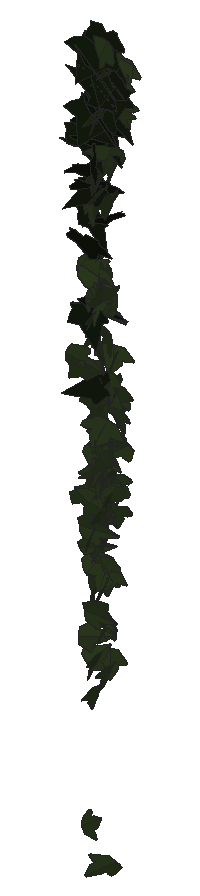
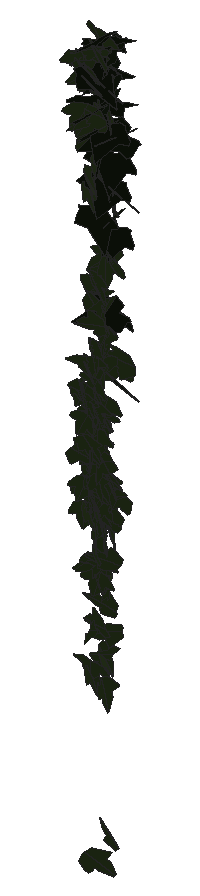
# SketchUp Ruby script. Lengths in inches.
U = 1.inch
M = Sketchup.active_model
def pt(a) = Geom::Point3d.new(a.map { |v| v * U })
def face(e, loops, mat)
  f = e.add_face(loops[0].map { |a| pt(a) })
  loops[1..].each { |l| e.add_face(l.map { |a| pt(a) }).erase! }
  f.material = f.back_material = mat if mat
  f
end
# faces: each face lists its corners as indices into pts; further lists are holes
def faces(e, pts, list, mat = nil) = list.each { |f| face(e, (f[0].is_a?(Array) ? f : [f]).map { |l| l.map { |i| pts[i] } }, mat) }
# xy, xz, yz: faces in a plane at the given z, y or x. An outline is a flat list of corners, or four numbers for a rectangle; further outlines are holes
def ring(l) = l.size == 4 ? [[l[0], l[1]], [l[2], l[1]], [l[2], l[3]], [l[0], l[3]]] : l.each_slice(2).to_a
def flat(e, list, mat, &to3) = list.each { |f| face(e, (f[0].is_a?(Array) ? f : [f]).map { |l| ring(l).map { |u, v| to3.(u, v) } }, mat) }
def xy(e, z, list, mat = nil) = flat(e, list, mat) { |x, y| [x, y, z] }
def xz(e, y, list, mat = nil) = flat(e, list, mat) { |x, z| [x, y, z] }
def yz(e, x, list, mat = nil) = flat(e, list, mat) { |y, z| [x, y, z] }
def lines(e, pts, list) = list.each { |a, b| e.add_line(pt(pts[a]), pt(pts[b])) }
# prism: a flat outline (further loops are holes) pulled along v
def prism(e, loops, v, mat = nil)
  f = face(e, loops, mat); d = Geom::Vector3d.new(v.map { |x| x * U })
  f.pushpull(f.normal.samedirection?(d) ? d.length : -d.length)
end
def box(e, o, s, mat = nil) = prism(e, [[o, [o[0] + s[0], o[1], o[2]], [o[0] + s[0], o[1] + s[1], o[2]], [o[0], o[1] + s[1], o[2]]]], [0, 0, s[2]], mat)
def at(x, y, z, deg = 0) = Geom::Transformation.translation(pt([x, y, z])) * Geom::Transformation.rotation(ORIGIN, Z_AXIS, deg.degrees)
def axes(o, x, y, z) = Geom::Transformation.new([*x, 0, *y, 0, *z, 0, *pt(o).to_a, 1])
def part(name) = M.definitions.add(name)
# library, detail: a bought-in or finely detailed component or shape, given as its bounding box
def library(name, o, s) = part(name).tap { |d| box(d.entities, o, s) }
def detail(e, o, s) = box(e.add_group.entities, o, s)
def put(e, d, t, mat = nil) = e.add_instance(d, t).tap { |i| i.material = mat if mat }
def group(e, t, mat = nil) = e.add_group.tap { |g| g.transformation = t; g.material = mat if mat }.entities
root = M.entities
M.materials.add("1026 AP 7946 SUNNY SIDE UP").color = [254, 231, 186]
M.materials.add("efeu1").color = [18, 25, 13]
M.materials.add("efeu2").color = [43, 57, 29]
c1 = part("ivyleaf_9")
p = [[1.54,2.16,1.25],[1.36,2.04,1.19],[-0.21,0.99,0.68],[-0.71,1.11,0.82],[-0.85,0.86,0.67],[-0.8,0.17,0.21],
  [-0.9,-0.01,0.1],[-0.67,-0.16,-0.02],[-0.08,-0.08,-0.05],[-0.03,-0.6,-0.4],[0.65,-0.88,-0.66],[0.83,-0.6,-0.49],
  [1.29,-0.42,-0.43],[1.8125,-0.07,-0.26],[1.21,0.44,0.15]]
faces(c1.entities,p,[[0,1,2,3,4,5,6,7,8,9,10,11,12,13,14]],"efeu1")
c2 = part("ivyleaf_10")
p = [[0,0.5,-0.03],[-0.0625,2.02,-0.43],[-0.19,2.01,-0.46],[-0.54,1.05,-0.29],[-0.52,0.625,-0.18],[-0.83,0.76,-0.28],
  [-1.16,0.64,-0.33],[-1.15,0.33,-0.24],[-0.77,-0.39,0.02],[-0.3,-0.51,0.16],[0.04,-0.48,0.23],[-0.02,2.01,-0.4375],
  [-0.06,2.01,-0.43],[0.04,-0.49,0.23],[0.67,-0.49,0.14],[1.38,0.36,-0.2],[1.375,0.51,-0.24],[0.81,0.65,-0.19],
  [0.62,0.59,-0.15],[0.6,1.09,-0.28],[0.5,1.23,-0.31]]
faces(c2.entities,p,[[0,1,2,3,4,5,6,7,8,9,10],[11,12,0,13,14,15,16,17,18,19,20]],"efeu2")
put(root,c1,axes([100.36,212.83,266.07],[0.33529,0.09717,-0.0854],[-0.10279,-0.05681,-0.24056],[-0.1732,0.22183,-0.02256]),"1026 AP 7946 SUNNY SIDE UP")
put(root,c2,axes([100.24,212.86,257.25],[-0.07001,-0.03539,0.18134],[0.17886,0.13359,0.05905],[-0.23398,0.1127,-0.00912]),"1026 AP 7946 SUNNY SIDE UP")
put(root,c2,axes([100.12,212.65,261.24],[-0.04534,-0.00324,-0.24949],[0.33942,-0.1109,-0.0256],[-0.17264,-0.21719,0.01519]),"1026 AP 7946 SUNNY SIDE UP")
put(root,c2,axes([100.23,212.86,251.5625],[0.15354,-0.11194,-0.14231],[0.15962,-0.09341,0.15206],[-0.22859,-0.14041,0.01059]),"1026 AP 7946 SUNNY SIDE UP")
put(root,c2,axes([100.43,212.78,258.9375],[0.16208,-0.18655,-0.02128],[-0.02221,0.01458,-0.21941],[0.2941,0.10391,-0.00484]),"1026 AP 7946 SUNNY SIDE UP")
put(root,c1,axes([100.23,212.74,265.85],[0.04431,-0.22984,-0.03374],[0.05092,0.03182,-0.24464],[0.38984,0.02197,0.03579]),"1026 AP 7946 SUNNY SIDE UP")
put(root,c2,axes([100.26,212.65,258.45],[-0.21018,-0.0282,-0.13125],[0.21154,-0.00791,-0.13329],[0.02448,-0.17381,0.02487]),"1026 AP 7946 SUNNY SIDE UP")
put(root,c1,axes([100.51,213.08,267.23],[0.001,0.16822,-0.15884],[0.00207,-0.15056,-0.18219],[-0.38323,-0.00038,-0.0014]),"1026 AP 7946 SUNNY SIDE UP")
put(root,c2,axes([100.24,213.1,262.17],[0.07325,-0.045,0.17694],[0.23261,-0.0942,-0.06684],[0.17607,0.14317,0.01469]),"1026 AP 7946 SUNNY SIDE UP")
put(root,c1,axes([100.45,212.58,265.3125],[0.16525,0.2139,-0.01562],[-0.01271,-0.01569,-0.25181],[-0.36408,0.09763,0.0017]),"1026 AP 7946 SUNNY SIDE UP")
put(root,c2,axes([100.375,212.94,260.22],[0.19343,-0.13157,0.05993],[0.05347,-0.04896,-0.18684],[0.23795,0.11796,-0.00673]),"1026 AP 7946 SUNNY SIDE UP")
put(root,c2,axes([100.375,212.87,262.48],[0.04091,0.22554,0.05224],[-0.00783,0.05028,-0.23335],[-0.36297,0.02433,0.01092]),"1026 AP 7946 SUNNY SIDE UP")
put(root,c1,axes([100.59,212.72,264.82],[-0.34947,0.07889,-0.04191],[0.04184,-0.04661,-0.23383],[-0.14435,-0.20451,0.0337]),"1026 AP 7946 SUNNY SIDE UP")
put(root,c2,axes([100.56,212.77,258.13],[-0.14192,0.09445,-0.14137],[-0.1209,0.11368,0.13565],[0.24956,0.10878,-0.01468]),"1026 AP 7946 SUNNY SIDE UP")
put(root,c2,axes([100.44,212.8,263.21],[-0.03803,-0.22151,-0.07694],[0.03725,0.07111,-0.22862],[0.36505,-0.03033,0.01531]),"1026 AP 7946 SUNNY SIDE UP")
put(root,c2,axes([100.47,212.72,266.15],[0.13869,-0.21441,-0.09491],[-0.02559,0.0913,-0.23756],[0.36529,0.0878,0.01939]),"1026 AP 7946 SUNNY SIDE UP")
put(root,c2,axes([100.67,212.75,258.93],[-0.11255,0.03358,0.18727],[-0.30155,-0.008,-0.07072],[-0.00733,-0.18649,0.03407]),"1026 AP 7946 SUNNY SIDE UP")
put(root,c1,axes([100.21,212.79,262.3],[0.32051,0.03421,0.09587],[0.1476,0.01981,-0.20512],[-0.06683,0.20784,0.00677]),"1026 AP 7946 SUNNY SIDE UP")
put(root,c1,axes([100.23,212.54,265.77],[0.37374,0.04867,0.08689],[0.11642,0.05727,-0.23701],[-0.10934,0.22733,0.04463]),"1026 AP 7946 SUNNY SIDE UP")
put(root,c2,axes([100.34,212.61,261.12],[-0.21705,-0.10609,-0.14613],[0.19367,0.07069,-0.17829],[0.19911,-0.18441,0.01412]),"1026 AP 7946 SUNNY SIDE UP")
put(root,c2,axes([100.49,212.89,258.88],[-0.15826,-0.18565,0.00326],[0.00844,-0.00771,-0.21743],[0.29188,-0.10044,0.00806]),"1026 AP 7946 SUNNY SIDE UP")
put(root,c2,axes([100.5,212.6,264.72],[0.11431,-0.19967,-0.11892],[-0.03891,0.11239,-0.21782],[0.35967,0.07562,0.01423]),"1026 AP 7946 SUNNY SIDE UP")
put(root,c2,axes([100.57,212.73,257.71],[-0.12137,0.1252,0.14101],[-0.18038,0.08393,-0.14784],[-0.24778,-0.12243,0.03855]),"1026 AP 7946 SUNNY SIDE UP")
put(root,c1,axes([100.41,212.54,263.81],[0.34902,0.0181,-0.10733],[-0.16564,-0.03169,-0.22029],[-0.05103,0.22664,-0.01899]),"1026 AP 7946 SUNNY SIDE UP")
put(root,c1,axes([100.42,212.73,264.84],[0.27748,0.14537,-0.04627],[-0.0441,-0.03858,-0.23442],[-0.25459,0.16513,-0.00982]),"1026 AP 7946 SUNNY SIDE UP")
put(root,c2,axes([100.54,213.01,262.99],[0.20632,-0.12535,-0.12004],[-0.10674,0.09227,-0.18483],[0.2628,0.13589,0.01917]),"1026 AP 7946 SUNNY SIDE UP")
put(root,c1,axes([100.31,212.85,264.15],[0.09917,-0.23323,-0.00491],[-0.00617,0.0025,-0.24886],[0.36672,0.06311,-0.00286]),"1026 AP 7946 SUNNY SIDE UP")
put(root,c2,axes([100.46,212.78,261.8],[0.01022,-0.21364,-0.08605],[0.0473,0.08243,-0.21747],[0.35688,-0.00481,0.03129]),"1026 AP 7946 SUNNY SIDE UP")
put(root,c1,axes([100.68,213.09,267.22],[-0.31077,0.12226,0.00258],[-0.02111,-0.01715,-0.23483],[-0.20647,-0.18227,0.02012]),"1026 AP 7946 SUNNY SIDE UP")
put(root,c2,axes([100.56,212.75,258.59],[-0.27272,-0.10409,0.04311],[-0.04072,-0.03892,-0.20763],[0.172,-0.17426,0.01919]),"1026 AP 7946 SUNNY SIDE UP")
put(root,c2,axes([100.56,212.96,259.79],[-0.32623,0.03364,0.03645],[-0.06096,-0.02101,-0.21491],[-0.04629,-0.20938,0.02615]),"1026 AP 7946 SUNNY SIDE UP")
put(root,c2,axes([100.53,212.61,256.62],[0.05783,-0.05067,-0.21146],[-0.00855,0.20776,-0.0527],[0.33189,0.01418,0.03549]),"1026 AP 7946 SUNNY SIDE UP")
put(root,c2,axes([100.51,212.74,262.19],[0.08681,-0.19783,0.05798],[0.01793,-0.05586,-0.2195],[0.3489,0.0521,-0.00314]),"1026 AP 7946 SUNNY SIDE UP")
put(root,c2,axes([100.5,212.76,260.39],[-0.31806,0.02153,-0.0272],[0.03891,-0.0241,-0.20097],[-0.04151,-0.18757,0.02]),"1026 AP 7946 SUNNY SIDE UP")
put(root,c2,axes([100.64,212.97,259.59],[-0.22626,-0.07226,0.11313],[-0.11797,-0.08882,-0.15871],[0.18407,-0.14575,0.03734]),"1026 AP 7946 SUNNY SIDE UP")
put(root,c2,axes([100.57,212.66,259.11],[0.07812,-0.16876,-0.09071],[-0.04925,0.07756,-0.18605],[0.31508,0.05397,-0.00659]),"1026 AP 7946 SUNNY SIDE UP")
put(root,c2,axes([100.51,212.81,261.49],[-0.1856,0.17454,0.00078],[-0.01694,-0.00807,-0.22018],[-0.29582,-0.10904,0.01212]),"1026 AP 7946 SUNNY SIDE UP")
put(root,c2,axes([100.68,213.1,259.67],[-0.2403,0.02295,0.11411],[-0.18458,-0.03124,-0.14825],[0.00144,-0.17424,0.03906]),"1026 AP 7946 SUNNY SIDE UP")
put(root,c1,axes([100.34,212.71,267.1],[0.33978,-0.12676,-0.03917],[-0.06132,0.00714,-0.25767],[0.19851,0.21917,-0.01255]),"1026 AP 7946 SUNNY SIDE UP")
put(root,c2,axes([100.71,212.93,258.8],[-0.24352,-0.0138,0.144],[-0.21332,-0.03966,-0.15902],[0.0577,-0.20487,0.01984]),"1026 AP 7946 SUNNY SIDE UP")
put(root,c2,axes([100.53,212.61,257.78],[0.11616,-0.18891,-0.00229],[0.00872,0.00341,-0.20884],[0.29692,0.0738,0.00703]),"1026 AP 7946 SUNNY SIDE UP")
put(root,c2,axes([100.51,212.79,261.71],[-0.14885,0.1889,0.01068],[-0.01244,0.00488,-0.22283],[-0.32067,-0.08787,0.00369]),"1026 AP 7946 SUNNY SIDE UP")
put(root,c1,axes([100.4,212.67,262.25],[-0.20148,-0.06412,-0.18126],[0.29207,0.01989,-0.13759],[0.0913,-0.20512,0.04015]),"1026 AP 7946 SUNNY SIDE UP")
put(root,c1,axes([100.62,212.85,264.16],[0.04967,0.21329,-0.0353],[-0.01558,-0.03482,-0.23092],[-0.36679,0.03036,0.00503]),"1026 AP 7946 SUNNY SIDE UP")
put(root,c2,axes([100.6,212.94,259.22],[-0.3082,0.07489,0.03653],[-0.06797,-0.01599,-0.21404],[-0.11081,-0.19847,0.02969]),"1026 AP 7946 SUNNY SIDE UP")
put(root,c1,axes([100.56,212.74,266.38],[-0.25884,-0.1792,0.02561],[-0.00352,-0.0326,-0.25149],[0.30743,-0.15125,0.01868]),"1026 AP 7946 SUNNY SIDE UP")
put(root,c2,axes([100.57,213.02,261.61],[0.20793,-0.14838,-0.10104],[-0.03675,0.10565,-0.19821],[0.27651,0.12562,0.04963]),"1026 AP 7946 SUNNY SIDE UP")
put(root,c2,axes([100.55,212.95,267.56],[0.25553,-0.19589,-0.00041],[-0.01636,-0.00956,-0.26186],[0.30758,0.16223,-0.01359]),"1026 AP 7946 SUNNY SIDE UP")
put(root,c2,axes([100.54,213.09,259.52],[0.09122,-0.16649,-0.05312],[0.04498,0.05701,-0.18122],[0.29042,0.04347,0.04476]),"1026 AP 7946 SUNNY SIDE UP")
put(root,c1,axes([100.79,212.58,260.88],[-0.31218,0.10579,0.04609],[-0.07383,0.00777,-0.22648],[-0.17833,-0.1884,0.01308]),"1026 AP 7946 SUNNY SIDE UP")
put(root,c2,axes([100.375,212.72,263.24],[0.27333,-0.05347,0.14211],[0.2091,-0.05196,-0.18215],[0.12579,0.20256,-0.006]),"1026 AP 7946 SUNNY SIDE UP")
put(root,c2,axes([100.38,212.77,264.52],[0.16742,-0.06672,0.21893],[0.24439,-0.14704,-0.12841],[0.25166,0.18718,-0.02093]),"1026 AP 7946 SUNNY SIDE UP")
put(root,c2,axes([100.54,212.93,257.46],[0.03884,-0.14276,0.15213],[0.05917,-0.1439,-0.14982],[0.31843,0.04415,0.00928]),"1026 AP 7946 SUNNY SIDE UP")
put(root,c1,axes([100.61,212.75,267.68],[-0.286,-0.17604,0.02969],[-0.00364,-0.04024,-0.25951],[0.28073,-0.17987,0.02688]),"1026 AP 7946 SUNNY SIDE UP")
put(root,c2,axes([100.45,212.76,257.13],[0.14241,0.15575,0.07555],[0.0744,0.05407,-0.1882],[-0.27912,0.09388,-0.01161]),"1026 AP 7946 SUNNY SIDE UP")
put(root,c2,axes([100.6,212.67,254.56],[-0.00997,-0.23049,-0.01947],[0.00768,0.01746,-0.23739],[0.36339,-0.00669,0.00448]),"1026 AP 7946 SUNNY SIDE UP")
put(root,c2,axes([100.34,213.11,262.14],[0.10099,0.00131,0.18023],[0.2795,0.03673,-0.06209],[-0.05951,0.17472,0.01425]),"1026 AP 7946 SUNNY SIDE UP")
put(root,c2,axes([100.56,213.02,260.43],[0.31079,-0.03823,-0.00996],[-0.0207,-0.01553,-0.19955],[0.0633,0.18263,-0.01638]),"1026 AP 7946 SUNNY SIDE UP")
put(root,c2,axes([100.64,212.97,267.04],[-0.19197,-0.1977,0.09896],[-0.01215,-0.1072,-0.23528],[0.34618,-0.11339,0.04662]),"1026 AP 7946 SUNNY SIDE UP")
put(root,c2,axes([100.52,212.86,258.36],[-0.28677,0.05931,-0.0818],[0.09657,-0.06374,-0.19394],[-0.12284,-0.18857,0.03849]),"1026 AP 7946 SUNNY SIDE UP")
put(root,c2,axes([100.63,212.71,266.39],[-0.01312,-0.24888,-0.02734],[-0.00692,0.02528,-0.25633],[0.39326,-0.00786,-0.00542]),"1026 AP 7946 SUNNY SIDE UP")
put(root,c1,axes([100.36,212.67,267.47],[0.22096,-0.19983,0.05888],[0.03742,-0.05432,-0.25581],[0.35104,0.13157,-0.0098]),"1026 AP 7946 SUNNY SIDE UP")
put(root,c2,axes([100.34,212.91,259.29],[0.1444,0.02951,0.1951],[0.29258,0.03586,-0.09859],[-0.07118,0.20724,-0.00945]),"1026 AP 7946 SUNNY SIDE UP")
put(root,c2,axes([100.43,212.56,255.64],[0.02374,-0.03529,-0.21241],[0.24299,0.14091,-0.01237],[0.22122,-0.151,0.03639]),"1026 AP 7946 SUNNY SIDE UP")
put(root,c2,axes([100.61,212.68,255.23],[0.0745,-0.22416,0.04769],[0.01115,-0.04712,-0.23629],[0.36014,0.04783,-0.00255]),"1026 AP 7946 SUNNY SIDE UP")
put(root,c2,axes([100.61,212.83,256.82],[-0.30128,0.01111,-0.01813],[0.02591,-0.02675,-0.18876],[-0.02291,-0.17628,0.02497]),"1026 AP 7946 SUNNY SIDE UP")
put(root,c2,axes([100.52,212.61,255.17],[0.12128,0.04858,-0.19863],[0.12404,0.18267,0.08087],[0.28745,-0.09932,0.04891]),"1026 AP 7946 SUNNY SIDE UP")
put(root,c2,axes([100.62,212.8,257.15],[-0.30963,-0.02386,-0.01274],[0.02756,-0.03677,-0.19309],[0.0356,-0.17903,0.0387]),"1026 AP 7946 SUNNY SIDE UP")
put(root,c1,axes([100.51,213.05,267.81],[-0.04211,-0.22509,0.04161],[-0.00942,-0.04145,-0.24301],[0.38852,-0.0254,-0.00138]),"1026 AP 7946 SUNNY SIDE UP")
put(root,c2,axes([100.58,212.72,263.5625],[0.20402,-0.1961,0.0693],[0.04045,-0.06484,-0.2422],[0.32404,0.13156,-0.0134]),"1026 AP 7946 SUNNY SIDE UP")
put(root,c2,axes([100.64,212.83,260.27],[-0.05629,-0.21802,-0.01507],[0.01029,0.0125,-0.22749],[0.34331,-0.03612,0.00435]),"1026 AP 7946 SUNNY SIDE UP")
put(root,c2,axes([100.7,212.625,260.92],[0.0966,-0.05898,-0.20841],[-0.08614,0.19084,-0.07543],[0.33309,0.06646,0.04094]),"1026 AP 7946 SUNNY SIDE UP")
put(root,c2,axes([100.58,212.97,260.83],[-0.27042,0.0638,-0.08937],[0.06479,-0.10748,-0.16578],[-0.16738,-0.14468,0.08022]),"1026 AP 7946 SUNNY SIDE UP")
put(root,c1,axes([100.74,213.09,267.07],[-0.33206,0.06591,-0.09323],[0.11649,-0.06699,-0.2181],[-0.14572,-0.20374,0.0381]),"1026 AP 7946 SUNNY SIDE UP")
put(root,c2,axes([100.64,212.75,259.99],[0.1608,-0.18738,0.0127],[-0.00063,-0.01546,-0.21985],[0.29538,0.10197,-0.00738]),"1026 AP 7946 SUNNY SIDE UP")
put(root,c1,axes([100.42,212.78,266.46],[0.19731,-0.21326,0.05946],[0.02451,-0.05905,-0.25472],[0.34704,0.12542,-0.01581]),"1026 AP 7946 SUNNY SIDE UP")
put(root,c1,axes([100.7,212.47,265.6],[0.10693,-0.04302,-0.26849],[-0.31791,0.16432,-0.08141],[0.2667,0.21312,0.01061]),"1026 AP 7946 SUNNY SIDE UP")
put(root,c2,axes([100.62,213.11,265.07],[0.14508,-0.17756,0.06874],[0.03898,-0.06274,-0.21174],[0.31951,0.08828,-0.00538]),"1026 AP 7946 SUNNY SIDE UP")
put(root,c1,axes([100.47,212.95,266],[0.06702,-0.23607,-0.05953],[0.02334,0.05973,-0.24548],[0.38095,0.03787,0.02552]),"1026 AP 7946 SUNNY SIDE UP")
put(root,c2,axes([100.66,212.77,264.75],[0.02038,-0.244,-0.00275],[0.00837,0.00157,-0.25165],[0.38358,0.01293,0.00564]),"1026 AP 7946 SUNNY SIDE UP")
put(root,c2,axes([100.4,212.97,255.95],[0.0969,0.01052,0.20769],[0.30784,-0.05427,-0.05907],[0.07703,0.20364,-0.02519]),"1026 AP 7946 SUNNY SIDE UP")
put(root,c2,axes([100.68,212.73,258.08],[0.12679,-0.18717,-0.0576],[-0.02747,0.05218,-0.2096],[0.30545,0.08239,0.00506]),"1026 AP 7946 SUNNY SIDE UP")
put(root,c2,axes([100.66,212.79,257.78],[0.01424,-0.19305,-0.0759],[0.02655,0.0731,-0.1977],[0.32321,0.0025,0.01959]),"1026 AP 7946 SUNNY SIDE UP")
put(root,c2,axes([100.68,212.84,259.64],[-0.01159,-0.18205,0.01798],[-0.00017,-0.01918,-0.1953],[0.31075,-0.0068,0.00057]),"1026 AP 7946 SUNNY SIDE UP")
put(root,c2,axes([100.68,212.71,258.18],[0.03291,-0.2112,0.00084],[0.00106,-0.00196,-0.21865],[0.3321,0.02093,0.00061]),"1026 AP 7946 SUNNY SIDE UP")
put(root,c2,axes([100.7,212.79,257.75],[0.09538,-0.13644,-0.14771],[-0.04098,0.14235,-0.1509],[0.30762,0.06127,0.0257]),"1026 AP 7946 SUNNY SIDE UP")
put(root,c2,axes([100.69,212.72,265.23],[-0.00139,-0.24332,0.02378],[-0.00032,-0.02446,-0.25081],[0.38453,-0.0009,-0.00012]),"1026 AP 7946 SUNNY SIDE UP")
put(root,c2,axes([100.63,212.88,260.01],[-0.17148,0.18172,-0.02763],[0.00846,-0.02922,-0.21824],[-0.28895,-0.1087,0.01001]),"1026 AP 7946 SUNNY SIDE UP")
put(root,c2,axes([100.63,212.74,259.66],[0.00019,0.21018,0.01882],[-0.01204,0.01707,-0.21628],[-0.33136,-0.0005,0.00787]),"1026 AP 7946 SUNNY SIDE UP")
put(root,c1,axes([100.61,213.07,266.65],[-0.17256,-0.19159,-0.03793],[0.06169,0.01778,-0.23058],[0.32419,-0.10537,0.02368]),"1026 AP 7946 SUNNY SIDE UP")
put(root,c2,axes([100.66,212.95,255.77],[0.0407,0.10043,-0.18382],[-0.04461,-0.17693,-0.10753],[-0.31964,0.03748,-0.0084]),"1026 AP 7946 SUNNY SIDE UP")
put(root,c2,axes([100.66,213.09,261.23],[0.13936,-0.16566,0.04137],[0.03169,-0.03629,-0.19844],[0.28788,0.08419,0.00182]),"1026 AP 7946 SUNNY SIDE UP")
put(root,c2,axes([100.83,212.75,251.01],[-0.15084,-0.0965,0.15959],[-0.15163,-0.12251,-0.14036],[0.2445,-0.1355,0.01141]),"1026 AP 7946 SUNNY SIDE UP")
put(root,c2,axes([100.7,212.875,259.4],[0.21587,-0.15358,-0.05876],[-0.03034,0.05761,-0.21053],[0.25533,0.13669,0.02466]),"1026 AP 7946 SUNNY SIDE UP")
put(root,c2,axes([100.71,212.9,254.92],[-0.00078,-0.21185,0.00821],[0.0004,-0.00917,-0.2183],[0.33342,-0.00049,0.00028]),"1026 AP 7946 SUNNY SIDE UP")
put(root,c2,axes([100.67,212.82,266.69],[0.17538,-0.22623,-0.02882],[0.03057,0.03906,-0.25717],[0.35688,0.10783,0.03619]),"1026 AP 7946 SUNNY SIDE UP")
put(root,c2,axes([100.63,213.1,261.33],[0.29306,0.07975,-0.00696],[0.00326,-0.02203,-0.20268],[-0.13595,0.17139,-0.01986]),"1026 AP 7946 SUNNY SIDE UP")
put(root,c2,axes([100.71,212.82,258.88],[0.06352,0.16131,-0.11024],[-0.09944,-0.09242,-0.17552],[-0.3113,0.06244,0.03358]),"1026 AP 7946 SUNNY SIDE UP")
put(root,c2,axes([100.6,212.6,258.38],[-0.11214,-0.1249,-0.16075],[0.1697,0.11257,-0.14738],[0.28236,-0.11726,0.02473]),"1026 AP 7946 SUNNY SIDE UP")
put(root,c2,axes([100.83,212.95,267.41],[0.26428,0.06824,-0.18473],[-0.24958,-0.08538,-0.18683],[-0.17049,0.23077,-0.01285]),"1026 AP 7946 SUNNY SIDE UP")
put(root,c2,axes([100.73,212.8,262.46],[-0.13777,-0.14387,0.12555],[0.01762,-0.13318,-0.16645],[0.31661,-0.05519,0.0639]),"1026 AP 7946 SUNNY SIDE UP")
put(root,c2,axes([100.74,212.95,258.64],[0.12267,-0.15914,-0.04441],[-0.04071,0.03234,-0.18645],[0.27531,0.07569,-0.00778]),"1026 AP 7946 SUNNY SIDE UP")
put(root,c2,axes([100.57,212.48,263.24],[0.09029,0.1495,0.17863],[0.1036,0.15326,-0.16768],[-0.36337,0.08084,-0.00342]),"1026 AP 7946 SUNNY SIDE UP")
put(root,c1,axes([100.55,213.1,266.35],[0.09425,-0.19911,-0.08343],[0.00173,0.0781,-0.2191],[0.36138,0.05156,0.02281]),"1026 AP 7946 SUNNY SIDE UP")
put(root,c2,axes([100.52,212.95,267.16],[-0.25668,-0.06793,-0.18768],[0.28999,0.01965,-0.17806],[0.095,-0.24354,0.03643]),"1026 AP 7946 SUNNY SIDE UP")
put(root,c2,axes([100.68,212.89,258.44],[-0.06785,0.17631,0.00301],[-0.00567,-0.00023,-0.19352],[-0.29924,-0.03997,0.00298]),"1026 AP 7946 SUNNY SIDE UP")
put(root,c2,axes([100.68,212.93,262.55],[0.27066,-0.1232,0.0277],[0.01408,-0.03396,-0.21494],[0.21381,0.15819,-0.02092]),"1026 AP 7946 SUNNY SIDE UP")
put(root,c2,axes([100.78,212.91,258.68],[-0.28466,-0.09556,0.04865],[-0.03862,-0.05425,-0.208],[0.16349,-0.1792,0.03558]),"1026 AP 7946 SUNNY SIDE UP")
put(root,c1,axes([101.03,212.58,266.9],[-0.09068,0.06253,0.25435],[-0.33767,0.1235,-0.0833],[-0.21431,-0.22104,0.02362]),"1026 AP 7946 SUNNY SIDE UP")
put(root,c2,axes([100.7,212.6875,267.78],[0.35655,-0.12,0.00498],[-0.00854,-0.02201,-0.26345],[0.18869,0.22575,-0.02133]),"1026 AP 7946 SUNNY SIDE UP")
put(root,c2,axes([100.61,213,255.13],[0.31353,-0.00839,0.05645],[0.08449,-0.02171,-0.20481],[0.02171,0.20565,-0.0181]),"1026 AP 7946 SUNNY SIDE UP")
put(root,c2,axes([100.71,212.8,256.98],[0.23937,0.10449,-0.05481],[-0.05883,-0.0413,-0.18803],[-0.18963,0.14471,-0.01085]),"1026 AP 7946 SUNNY SIDE UP")
put(root,c2,axes([100.46,212.5625,257.87],[-0.06952,0.00868,0.22828],[0.34088,0.04901,0.04288],[-0.07302,0.22053,-0.01716]),"1026 AP 7946 SUNNY SIDE UP")
put(root,c2,axes([100.59,213.07,266.25],[0.32708,0.0566,0.09255],[0.11387,0.06864,-0.209],[-0.13204,0.1994,0.04901]),"1026 AP 7946 SUNNY SIDE UP")
put(root,c2,axes([100.76,212.93,258.23],[0.01817,-0.20992,0.02189],[0.0007,-0.02245,-0.21672],[0.33196,0.01154,-0.00074]),"1026 AP 7946 SUNNY SIDE UP")
put(root,c2,axes([100.86,213.11,259.41],[0.1134,0.08523,-0.14874],[-0.22226,-0.06327,-0.10897],[-0.16748,0.14167,0.04391]),"1026 AP 7946 SUNNY SIDE UP")
put(root,c2,axes([100.62,212.86,259.69],[-0.26117,0.0209,0.11734],[0.18444,-0.01236,0.16604],[0.04108,0.18834,0.00054]),"1026 AP 7946 SUNNY SIDE UP")
put(root,c2,axes([100.68,213.11,266.39],[-0.29468,-0.11542,-0.07506],[0.14075,-0.00395,-0.21755],[0.17928,-0.18661,0.04743]),"1026 AP 7946 SUNNY SIDE UP")
put(root,c2,axes([100.74,212.7,262.63],[-0.09209,-0.21991,-0.07428],[-0.04627,-0.0654,0.23378],[-0.36033,0.0646,-0.01104]),"1026 AP 7946 SUNNY SIDE UP")
put(root,c2,axes([100.71,213.1,260.11],[-0.2537,0.08851,-0.04189],[0.0428,-0.03608,-0.18548],[-0.15943,-0.15052,0.01688]),"1026 AP 7946 SUNNY SIDE UP")
put(root,c2,axes([100.71,213.11,267.23],[0.31917,-0.10491,0.0218],[0.02358,-0.01965,-0.23052],[0.18034,0.18825,-0.00844]),"1026 AP 7946 SUNNY SIDE UP")
put(root,c2,axes([100.76,212.84,258.81],[-0.02902,-0.19305,-0.01183],[0.03478,0.0067,-0.20631],[0.32618,-0.01789,0.02094]),"1026 AP 7946 SUNNY SIDE UP")
put(root,c2,axes([100.79,212.65,256.77],[0.10645,-0.20723,-0.02721],[-0.02689,0.02093,-0.22425],[0.32716,0.06915,-0.00958]),"1026 AP 7946 SUNNY SIDE UP")
put(root,c2,axes([100.8,212.76,267.28],[-0.03085,-0.2537,-0.04742],[0.00003,0.04472,-0.26186],[0.40504,-0.01933,-0.00359]),"1026 AP 7946 SUNNY SIDE UP")
put(root,c2,axes([100.63,212.86,260.58],[0.16083,-0.09939,0.15064],[0.17654,-0.09688,-0.14822],[0.2354,0.14056,0.00823]),"1026 AP 7946 SUNNY SIDE UP")
put(root,c2,axes([100.73,212.64,259.3125],[-0.02693,-0.16461,-0.14332],[0.08464,0.13092,-0.16677],[0.32718,-0.04742,0.03135]),"1026 AP 7946 SUNNY SIDE UP")
put(root,c2,axes([100.64,212.68,258.97],[0.17209,-0.07589,0.15447],[0.16405,-0.11029,-0.13542],[0.22472,0.13862,-0.01943]),"1026 AP 7946 SUNNY SIDE UP")
put(root,c2,axes([100.51,212.6,256.125],[-0.0408,0.00263,0.20633],[0.32688,0.00791,0.02571],[-0.01278,0.19402,-0.00114]),"1026 AP 7946 SUNNY SIDE UP")
put(root,c2,axes([100.78,213.07,260.74],[0.1062,-0.17592,-0.05092],[-0.00463,0.04697,-0.19877],[0.30834,0.0613,0.01456]),"1026 AP 7946 SUNNY SIDE UP")
put(root,c2,axes([100.76,212.8,256.95],[0.28545,0.06143,-0.03898],[-0.06725,0.00031,-0.1911],[-0.10169,0.17222,0.01696]),"1026 AP 7946 SUNNY SIDE UP")
put(root,c2,axes([100.76,212.66,260.04],[0.35188,0.00864,-0.03624],[-0.05635,-0.01695,-0.22174],[-0.01908,0.20937,-0.0135]),"1026 AP 7946 SUNNY SIDE UP")
put(root,c2,axes([100.8,212.6875,260.79],[0.13295,-0.20033,-0.02147],[-0.02043,0.0159,-0.22384],[0.31587,0.08535,-0.00544]),"1026 AP 7946 SUNNY SIDE UP")
put(root,c2,axes([100.84,212.83,258.64],[-0.17783,-0.15155,0.09182],[-0.03908,-0.09214,-0.19258],[0.27437,-0.11135,0.03208]),"1026 AP 7946 SUNNY SIDE UP")
put(root,c2,axes([100.82,212.74,265.625],[-0.22839,-0.18829,0.07025],[-0.00325,-0.0841,-0.24049],[0.31544,-0.13719,0.04839]),"1026 AP 7946 SUNNY SIDE UP")
put(root,c2,axes([100.77,212.93,259.06],[-0.01631,-0.07559,0.16969],[0.04946,-0.15821,-0.08061],[0.2955,0.02231,0.02286]),"1026 AP 7946 SUNNY SIDE UP")
put(root,c2,axes([100.75,213.01,258.77],[-0.21642,-0.11414,-0.05566],[0.08791,0.01732,-0.1816],[0.19278,-0.13603,0.02032]),"1026 AP 7946 SUNNY SIDE UP")
put(root,c2,axes([100.8,212.79,258.56],[0.05337,-0.19667,-0.08061],[0.00576,0.07866,-0.2045],[0.33213,0.03024,0.0165]),"1026 AP 7946 SUNNY SIDE UP")
put(root,c1,axes([100.72,212.78,267.37],[-0.11971,-0.24495,0.03227],[-0.00285,-0.03368,-0.26431],[0.38857,-0.07571,0.00801]),"1026 AP 7946 SUNNY SIDE UP")
put(root,c2,axes([100.8125,213.05,260.53],[0.29126,-0.07396,-0.04532],[-0.07148,0.00666,-0.19963],[0.12484,0.17637,-0.00856]),"1026 AP 7946 SUNNY SIDE UP")
put(root,c2,axes([100.83,212.81,264.68],[-0.00583,-0.24233,0.00362],[0.00473,-0.00493,-0.24969],[0.38109,-0.00365,0.00316]),"1026 AP 7946 SUNNY SIDE UP")
put(root,c2,axes([100.83,212.93,258.2],[-0.23512,-0.11824,-0.01234],[0.02795,-0.00395,-0.19447],[0.19948,-0.13881,0.0127]),"1026 AP 7946 SUNNY SIDE UP")
put(root,c2,axes([100.82,212.95,267.38],[0.32801,0.1312,-0.06918],[-0.10395,-0.02216,-0.25348],[-0.20773,0.21826,0.0176]),"1026 AP 7946 SUNNY SIDE UP")
put(root,c1,axes([100.58,212.94,267.03],[0.06302,-0.12941,0.22005],[0.1313,-0.19773,-0.14023],[0.37115,0.09192,0.01225]),"1026 AP 7946 SUNNY SIDE UP")
put(root,c2,axes([100.79,213.01,260.65],[-0.28523,0.06905,-0.03699],[0.04454,-0.02902,-0.19408],[-0.124,-0.16925,0.01536]),"1026 AP 7946 SUNNY SIDE UP")
